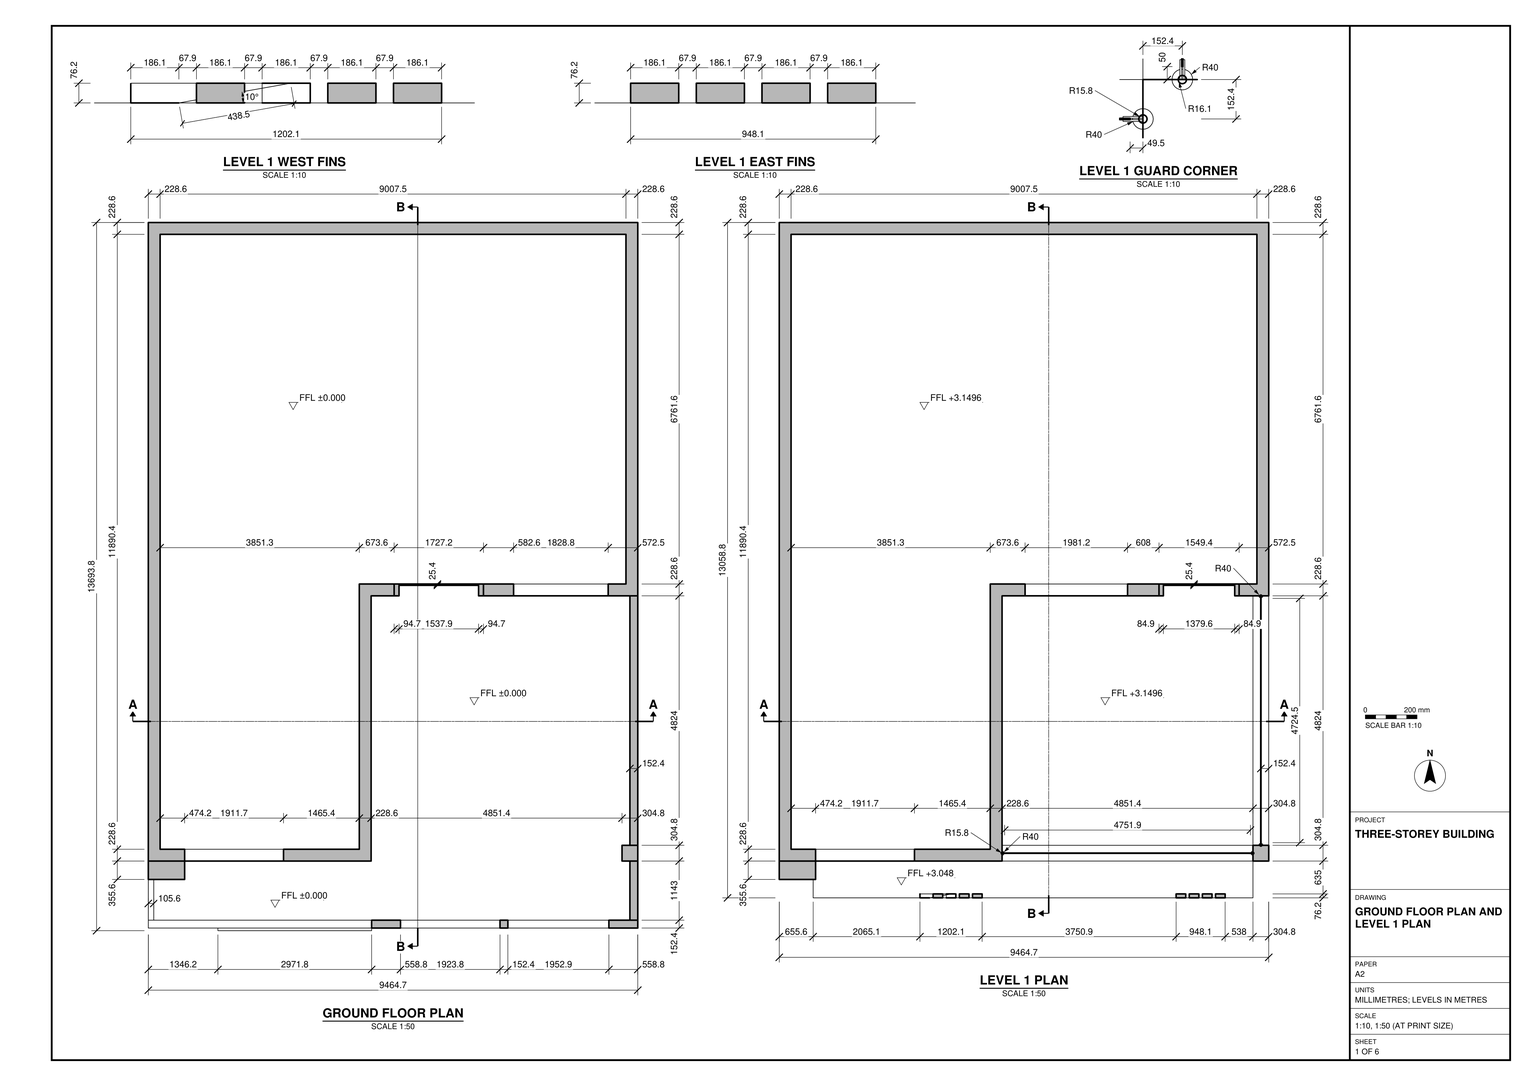
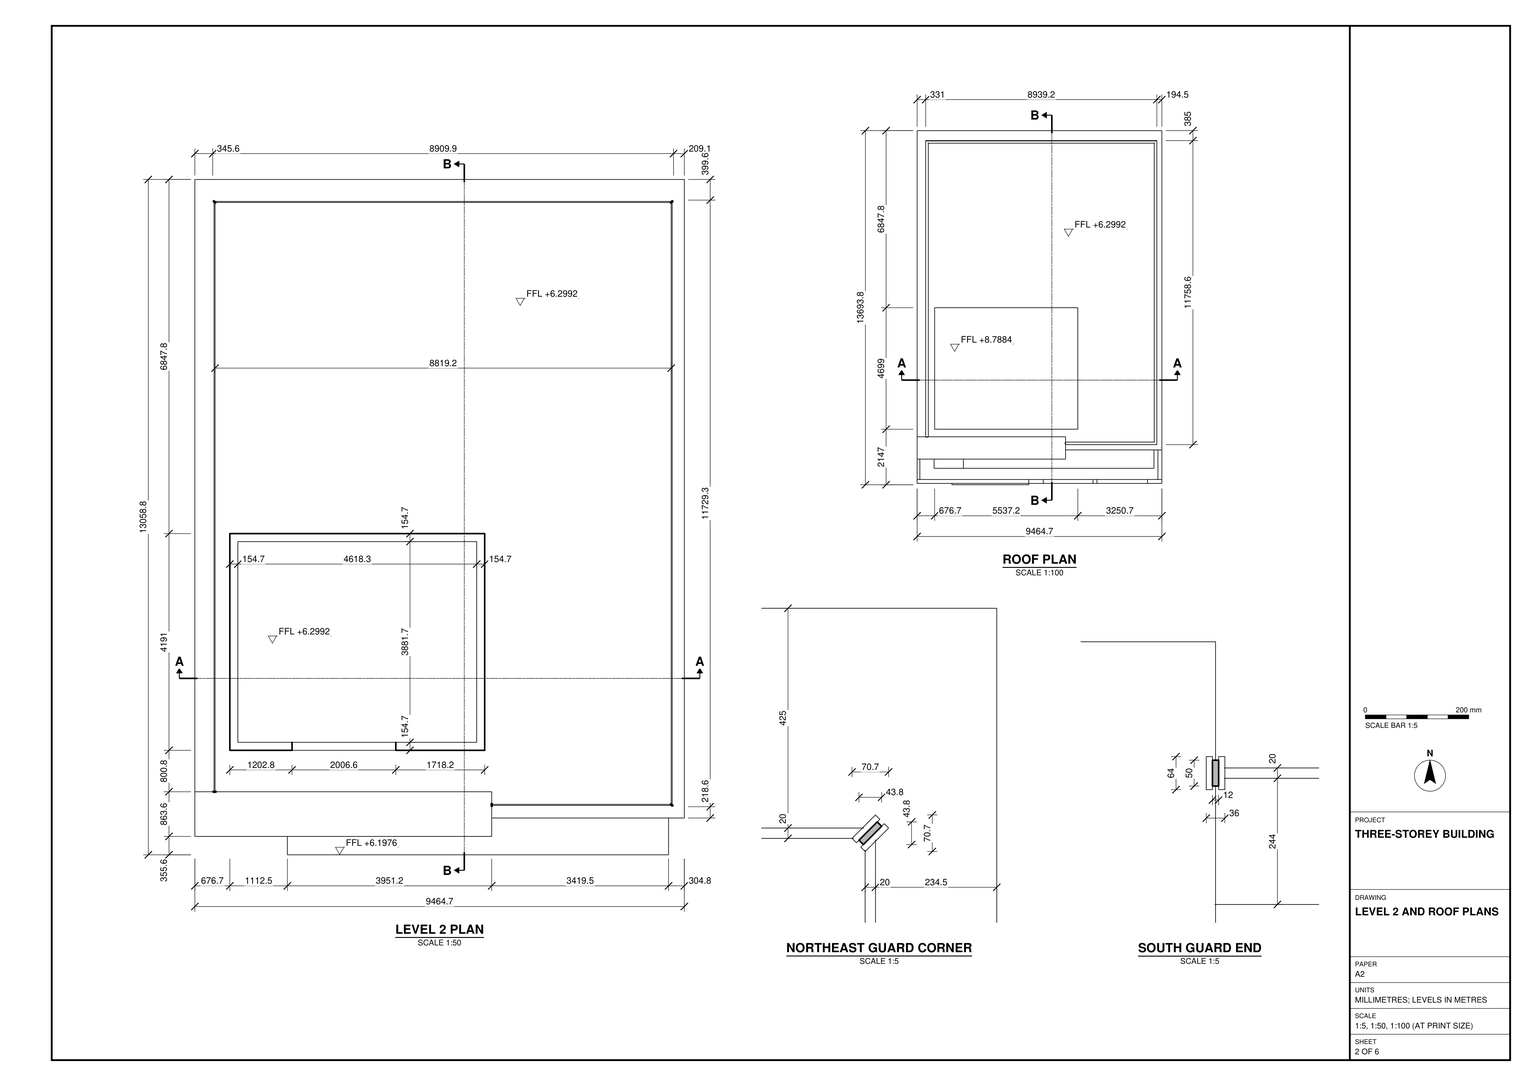
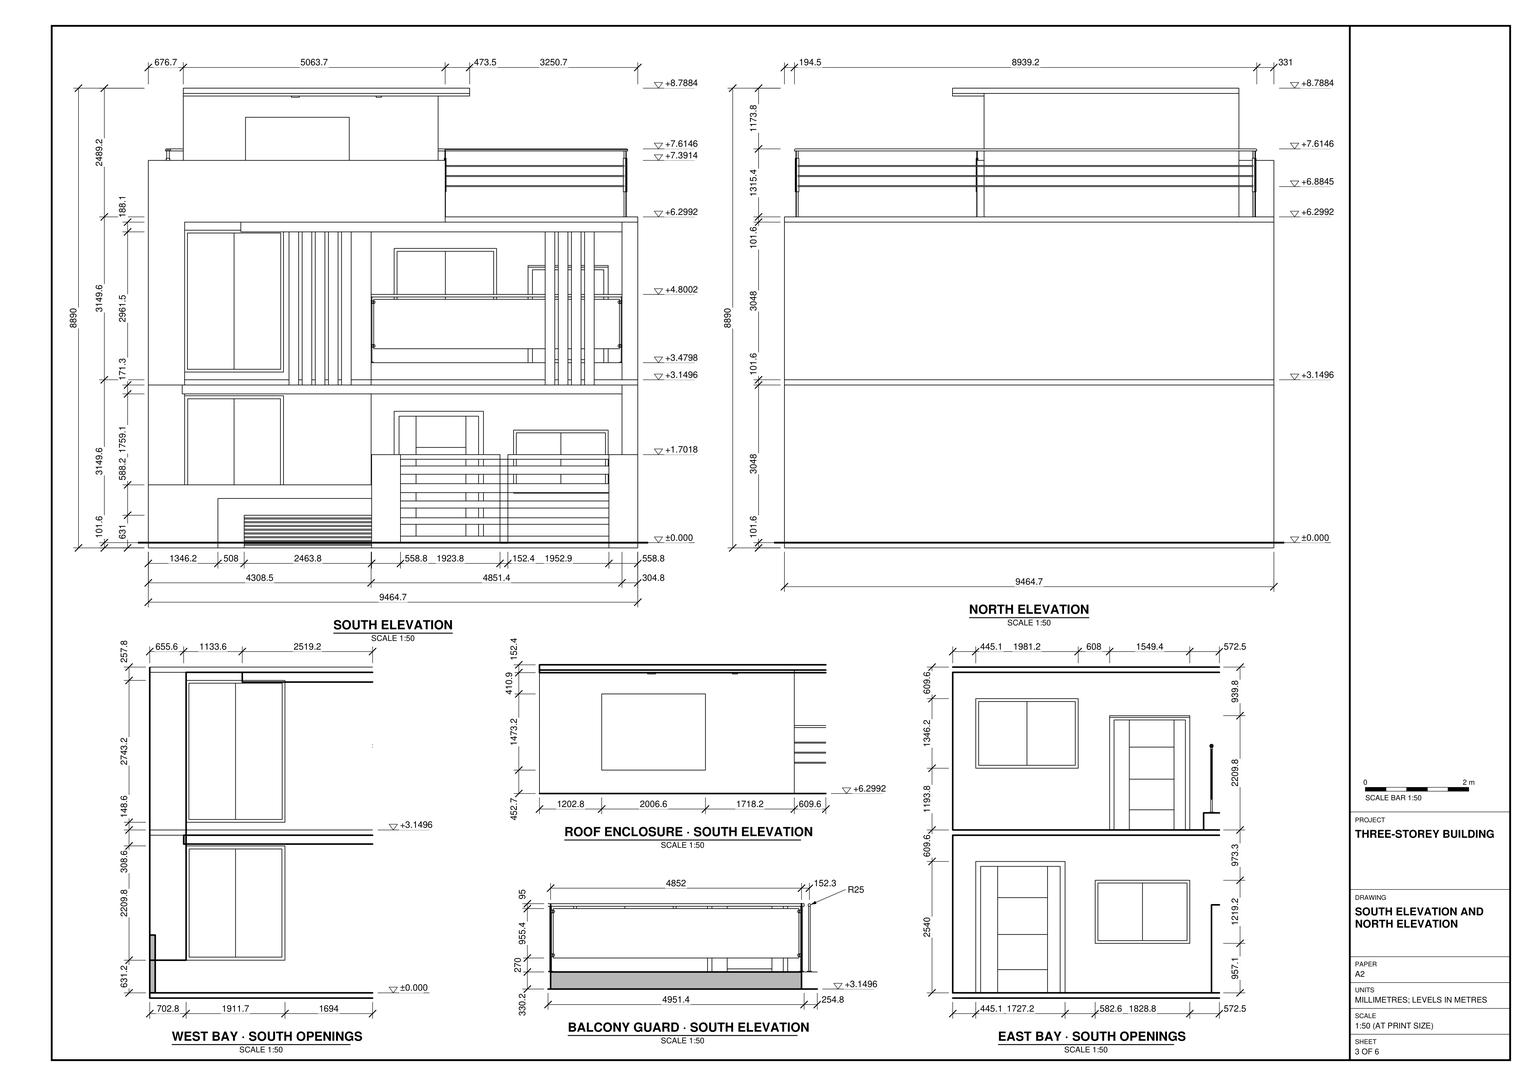
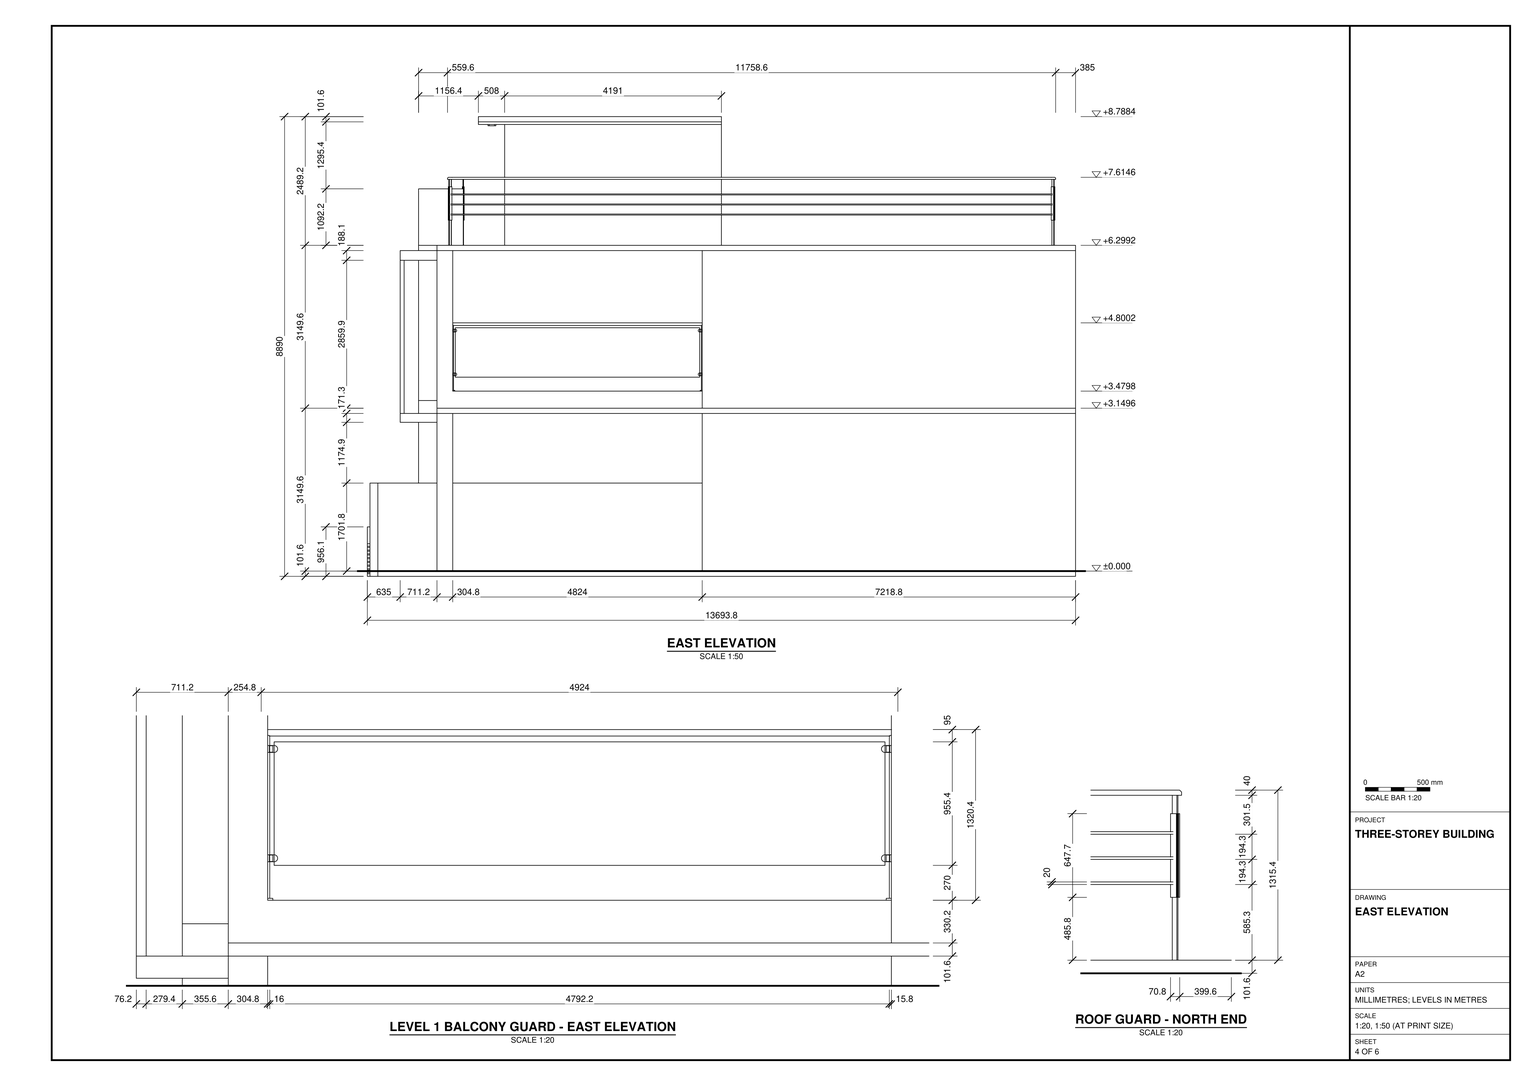
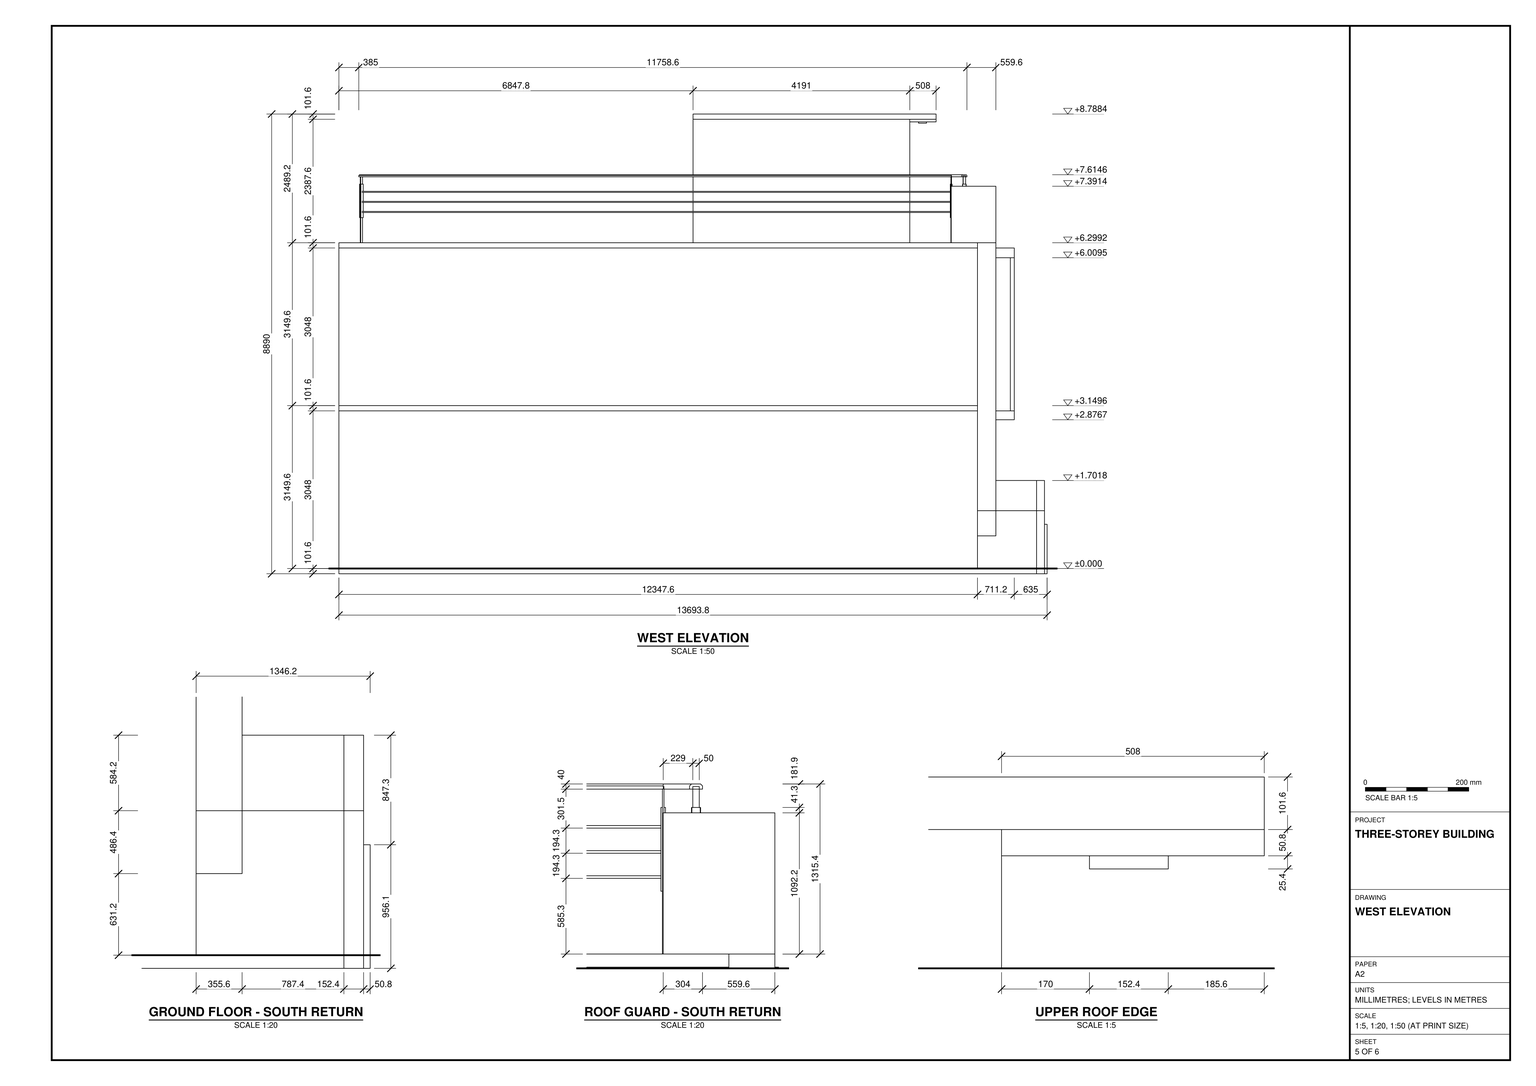
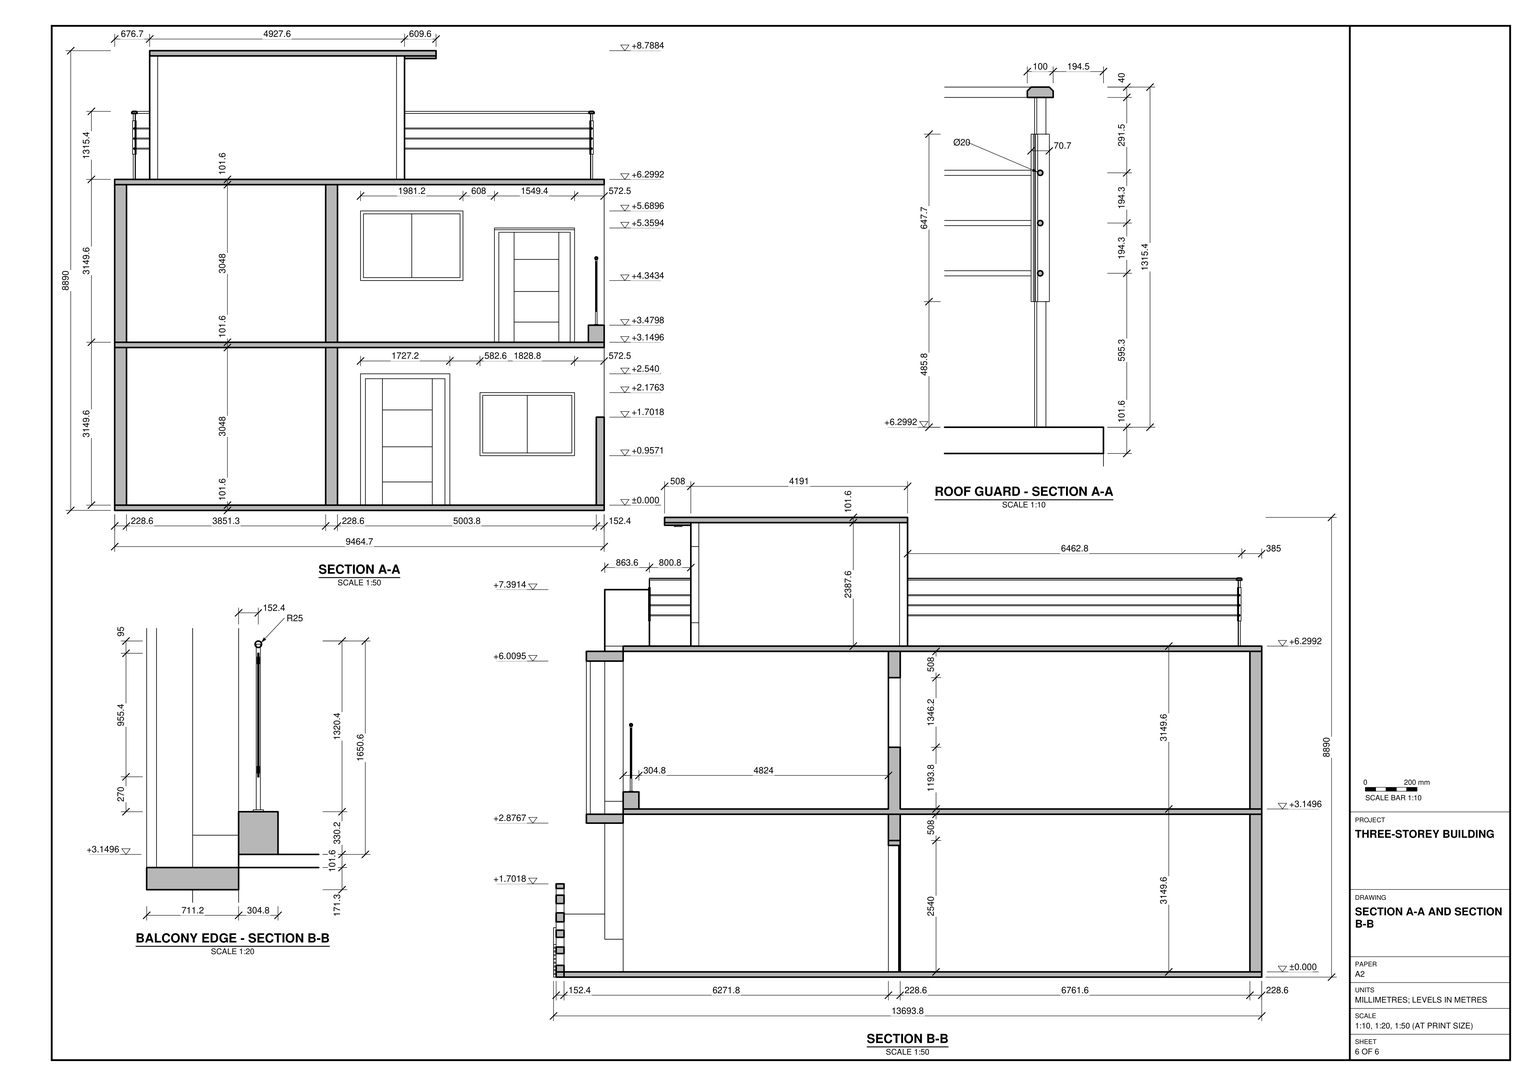
Build the three-storey building in SketchUp from task_files/diagram_01.pdf. Work in millimetres. The overall dimensions are 9464.7 mm east–west, 13693.8 mm north–south and 8890 mm high. Set the ground floor at 0 mm, level 1 at +3149.6 mm and level 2 at +6299.2 mm.

Use the floor plans to lay out the full-width north end, the projecting southwest bay and the recessed southeast bay. Model the floor slabs, the 228.6 mm main walls and the thinner walls where indicated. Keep the north wall uninterrupted by openings. On the south side, fit the tall paired window units in the west bay and the doors and windows in the recessed wall. Follow the elevations for their sill and head heights. Model the low front wall and horizontal slatted panels at ground level. At level 1, include the balcony guard, its corner return and the two distinct sets of vertical fins.

At level 2, form the open terrace with its parapet and rails. Place the smaller walled enclosure toward the southwest, with its south-facing opening and projecting flat roof. Keep walls, slabs, roof elements and each furniture or joinery piece shown in separate groups or components, and use components for repeated parts. Any decor or loose items shown may be represented by suitable library components. Save one SketchUp model as output_files/three_storey_building_with_a_balcony_and_roof_terrace.skp.

# SketchUp Ruby script. Lengths in millimetres.
U = 1.mm
M = Sketchup.active_model
def pt(a) = Geom::Point3d.new(a.map { |v| v * U })
def face(e, loops, mat)
  f = e.add_face(loops[0].map { |a| pt(a) })
  loops[1..].each { |l| e.add_face(l.map { |a| pt(a) }).erase! }
  f.material = f.back_material = mat if mat
  f
end
# faces: each face lists its corners as indices into pts; further lists are holes
def faces(e, pts, list, mat = nil) = list.each { |f| face(e, (f[0].is_a?(Array) ? f : [f]).map { |l| l.map { |i| pts[i] } }, mat) }
# xy, xz, yz: faces in a plane at the given z, y or x. An outline is a flat list of corners, or four numbers for a rectangle; further outlines are holes
def ring(l) = l.size == 4 ? [[l[0], l[1]], [l[2], l[1]], [l[2], l[3]], [l[0], l[3]]] : l.each_slice(2).to_a
def flat(e, list, mat, &to3) = list.each { |f| face(e, (f[0].is_a?(Array) ? f : [f]).map { |l| ring(l).map { |u, v| to3.(u, v) } }, mat) }
def xy(e, z, list, mat = nil) = flat(e, list, mat) { |x, y| [x, y, z] }
def xz(e, y, list, mat = nil) = flat(e, list, mat) { |x, z| [x, y, z] }
def yz(e, x, list, mat = nil) = flat(e, list, mat) { |y, z| [x, y, z] }
def lines(e, pts, list) = list.each { |a, b| e.add_line(pt(pts[a]), pt(pts[b])) }
# prism: a flat outline (further loops are holes) pulled along v
def prism(e, loops, v, mat = nil)
  f = face(e, loops, mat); d = Geom::Vector3d.new(v.map { |x| x * U })
  f.pushpull(f.normal.samedirection?(d) ? d.length : -d.length)
end
def box(e, o, s, mat = nil) = prism(e, [[o, [o[0] + s[0], o[1], o[2]], [o[0] + s[0], o[1] + s[1], o[2]], [o[0], o[1] + s[1], o[2]]]], [0, 0, s[2]], mat)
def at(x, y, z, deg = 0) = Geom::Transformation.translation(pt([x, y, z])) * Geom::Transformation.rotation(ORIGIN, Z_AXIS, deg.degrees)
def axes(o, x, y, z) = Geom::Transformation.new([*x, 0, *y, 0, *z, 0, *pt(o).to_a, 1])
def part(name) = M.definitions.add(name)
# library, detail: a bought-in or finely detailed component or shape, given as its bounding box
def library(name, o, s) = part(name).tap { |d| box(d.entities, o, s) }
def detail(e, o, s) = box(e.add_group.entities, o, s)
def put(e, d, t, mat = nil) = e.add_instance(d, t).tap { |i| i.material = mat if mat }
def group(e, t, mat = nil) = e.add_group.tap { |g| g.transformation = t; g.material = mat if mat }.entities
root = M.entities
M.materials.add("[Cladding Siding Tan]").color = [162, 126, 95]
M.materials.add("[Color B07]").color = [153, 38, 0]
M.materials.add("[Color C07]").color = [153, 76, 0]
M.materials.add("[Color E04]").color = [255, 255, 50]
M.materials.add("[Color M06]").color = [86, 86, 86]
M.materials.add("[Color M09]").color = [0, 0, 0]
M.materials.add("[Wood Veneer 01]").color = [120, 70, 37]
M.materials.add("[Wood Veneer 02]").color = [190, 128, 91]
c1 = library("Group\#4",[0,0,0],[4951.4,80,1320.4])
c2 = library("Group\#11",[0,0,0],[80,4924,1320.4])
c3 = library("Group\#7",[0,0,0],[8939.2,11758.6,730.1])
c4 = part("Ploe")
box(c4.entities,[5734.4,229,6400.8],[12,50,1295.4])
box(c4.entities,[5746.4,222,6886.6],[12,64,647.7],"[Wood Veneer 02]")
box(c4.entities,[5722.4,222,6886.6],[12,64,647.7],"[Wood Veneer 02]")
c5 = part("Group8\#1")
put(c5.entities,c4,at(0,0,0))
put(c5.entities,c4,at(5340.7,-3984.7,0,45))
put(c5.entities,c4,at(4981.5,15792.1,0,-45))
put(c5.entities,c4,at(4260.5,16151.3,0,-135))
put(c5.entities,c4,at(127,6248.4,0,-90))
c6 = part("Horizontal slat panel")
box(c6.entities,[0,-50.8,0],[2463.8,50.8,50.3])
box(c6.entities,[0,-50.8,-72.6],[2463.8,50.8,50.3])
box(c6.entities,[0,-50.8,-145.2],[2463.8,50.8,50.3])
box(c6.entities,[0,-50.8,-217.8],[2463.8,50.8,50.4])
box(c6.entities,[0,-50.8,-290.3],[2463.8,50.8,50.3])
box(c6.entities,[0,-50.8,-362.9],[2463.8,50.8,50.3])
box(c6.entities,[0,-50.8,-435.5],[2463.8,50.8,50.3])
box(c6.entities,[0,-50.8,-508.1],[2463.8,50.8,50.3])
box(c6.entities,[0,-50.8,-580.7],[2463.8,50.8,50.3])
c7 = part("Group\#10")
xy(c7.entities,0,[[0,0,0,228.6,1727.2,228.6,1727.2,0,1632.5,0,1632.5,203.2,94.7,203.2,94.7,0]],"[Wood Veneer 01]")
xy(c7.entities,2445.3,[[94.7,0,1632.5,203.2]],"[Wood Veneer 01]")
xy(c7.entities,2540,[[0,0,1727.2,228.6]],"[Wood Veneer 01]")
xz(c7.entities,0,[[0,0,94.7,0,94.7,2445.3,1632.5,2445.3,1632.5,0,1727.2,0,1727.2,2540,0,2540]],"[Wood Veneer 01]")
xz(c7.entities,203.2,[[94.7,0,423.7,2445.3],[423.7,0,1387.9,448.6],[1387.9,0,1632.5,2445.3],[423.7,448.6,1387.9,1128.7],[423.7,1128.7,1387.9,1841.3],
  [423.7,1841.3,1387.9,2445.3]],"[Wood Veneer 01]")
xz(c7.entities,228.6,[[0,0,1727.2,2540]],"[Wood Veneer 01]")
yz(c7.entities,0,[[0,0,228.6,2540]],"[Wood Veneer 01]")
yz(c7.entities,94.7,[[0,0,203.2,2445.3]],"[Wood Veneer 01]")
yz(c7.entities,1632.5,[[0,0,203.2,2445.3]],"[Wood Veneer 01]")
yz(c7.entities,1727.2,[[0,0,228.6,2540]],"[Wood Veneer 01]")
box(root,[3482.7,635,3149.6],[186.1,76.2,2961.5],"[Color M06]")
box(root,[3736.7,635,3149.6],[186.1,76.2,2961.5],"[Color M06]")
box(root,[7673.7,635,3149.6],[186.1,76.2,2961.5],"[Color M06]")
box(root,[7927.7,635,3149.6],[186.1,76.2,2961.5],"[Color M06]")
box(root,[8181.7,635,3149.6],[186.1,76.2,2961.5],"[Color M06]")
box(root,[8435.7,635,3149.6],[186.1,76.2,2961.5],"[Color M06]")
prism(root,[[[9464.7,1651,101.6],[9464.7,2870.2,101.6],[9464.7,6475,101.6],[9464.7,6475,1803.4],[9464.7,1651,1803.4]]],[-152.4,0,0])
xy(root,0,[[4318,50.8,8905.9,203.2],[8905.9,50.8,9464.7,203.2]])
xy(root,88.4,[[6800.6,50.8,6953,203.2]])
xy(root,100.3,[[4876.8,50.8,8905.9,203.2]])
xy(root,101.6,[[0,203.2,105.6,1346.2],[9312.3,203.2,9464.7,1346.2]])
xy(root,227.5,[[4876.8,50.8,8905.9,203.2]],"[Color M06]")
xy(root,455.6,[[4876.8,50.8,8905.9,203.2]],"[Color M06]")
xy(root,582.2,[[4876.8,50.8,8905.9,203.2]],"[Color M06]")
xy(root,732.8,[[0,990.6,702.8,1346.2]])
xy(root,770.3,[[4876.8,50.8,8905.9,203.2]],"[Color M06]")
xy(root,907.6,[[4876.8,50.8,8905.9,203.2]],"[Color M06]")
xy(root,1069.1,[[4876.8,50.8,8905.9,203.2]],"[Color M06]")
xy(root,1219.2,[[0,203.2,105.6,1346.2]])
xy(root,1242.2,[[4876.8,50.8,8905.9,203.2]],"[Color M06]")
xy(root,1423.5,[[4876.8,50.8,8905.9,203.2]],"[Color M06]")
xy(root,1584.5,[[4876.8,50.8,8905.9,203.2]],"[Color M06]")
xy(root,1714,[[4876.8,50.8,6800.6,203.2],[6953,50.8,8905.9,203.2]],"[Color M06]")
xy(root,1714,[[6800.6,50.8,6953,203.2]],"[Color M09]")
xy(root,1803.4,[[4318,50.8,4876.8,203.2],[8905.9,50.8,9464.7,203.2],[9312.3,203.2,9464.7,1346.2]])
xy(root,1803.4,[[4876.8,50.8,6800.6,203.2],[6953,50.8,8905.9,203.2]],"[Color M06]")
xy(root,3149.6,[[2720.7,635,2720.7,711.2,2974.7,711.2,2974.7,647,2906.8,635],[2974.7,635,2974.7,647,3160.8,679.8,3160.8,635],[3228.7,635,3228.7,691.8,3338.6,711.2,3414.8,711.2,3414.8,635],[2974.7,647,2974.7,711.2,3160.8,711.2,3160.8,679.8],[3160.8,679.8,3160.8,711.2,3228.7,711.2,3228.7,691.8],
  [3228.7,691.8,3228.7,711.2,3338.6,711.2]],"[Color M06]")
xy(root,6111.1,[[2720.7,635,2906.8,635,2974.7,647,2974.7,711.2,2720.7,711.2],[2974.7,635,3160.8,635,3160.8,679.8,2974.7,647],[3228.7,635,3414.8,635,3414.8,711.2,3338.6,711.2,3228.7,691.8],[2974.7,647,3160.8,679.8,3160.8,711.2,2974.7,711.2],[3160.8,679.8,3228.7,691.8,3228.7,711.2,3160.8,711.2],
  [3228.7,691.8,3338.6,711.2,3228.7,711.2]],"[Color M06]")
xy(root,6299.2,[[702.8,990.6,5740.4,1346.2]])
xy(root,6400.8,[[0,1346.2,5740.4,1854.2],[[676.7,2655,5604.3,6846],[831.4,2809.6,5449.7,6691.3]],[831.4,2809.6,5449.7,6691.3]])
xy(root,6853.5,[[1879.5,2655,3886.1,2809.6]])
xy(root,7493,[[0,990.6,5740.4,1854.2]])
xy(root,8326.7,[[1879.5,2655,3886.1,2809.6]])
xy(root,8712.2,[[2843.1,2332.6,2823.4,2335.2,2805,2342.8,2789.2,2354.9,2777.1,2370.7,2769.5,2389.1,2766.9,2408.8,2769.5,2428.5,2777.1,2446.9,2789.2,2462.7,2805,2474.8,2823.4,2482.4,2843.1,2485,2862.8,2482.4,2881.2,2474.8,2897,2462.7,2909.1,2446.9,2916.7,2428.5,2919.3,2408.8,2916.7,2389.1,2909.1,2370.7,2897,2354.9,2881.2,2342.8,2862.8,2335.2],[4456.2,2356.9,4443,2358.6,4430.8,2363.7,4420.3,2371.8,4412.2,2382.3,4407.1,2394.6,4405.4,2407.7,4407.1,2420.9,4412.2,2433.1,4420.3,2443.6,4430.8,2451.7,4443,2456.8,4456.2,2458.5,4469.3,2456.8,4481.6,2451.7,4492.1,2443.6,4500.2,2433.1,4505.2,2420.9,4507,2407.7,4505.2,2394.6,4500.2,2382.3,4492.1,2371.8,4481.6,2363.7,4469.3,2358.6]],"[Color E04]")
xy(root,8737.6,[[[676.7,2147,676.7,2655,5604.3,2655,5604.3,6846,6213.9,6846,6213.9,2147],[2843.1,2332.6,2862.8,2335.2,2881.2,2342.8,2897,2354.9,2909.1,2370.7,2916.7,2389.1,2919.3,2408.8,2916.7,2428.5,2909.1,2446.9,2897,2462.7,2881.2,2474.8,2862.8,2482.4,2843.1,2485,2823.4,2482.4,2805,2474.8,2789.2,2462.7,2777.1,2446.9,2769.5,2428.5,2766.9,2408.8,2769.5,2389.1,2777.1,2370.7,2789.2,2354.9,2805,2342.8,2823.4,2335.2],[4456.2,2356.9,4469.3,2358.6,4481.6,2363.7,4492.1,2371.8,4500.2,2382.3,4505.2,2394.6,4507,2407.7,4505.2,2420.9,4500.2,2433.1,4492.1,2443.6,4481.6,2451.7,4469.3,2456.8,4456.2,2458.5,4443,2456.8,4430.8,2451.7,4420.3,2443.6,4412.2,2433.1,4407.1,2420.9,4405.4,2407.7,4407.1,2394.6,4412.2,2382.3,4420.3,2371.8,4430.8,2363.7,4443,2358.6]]],"[Color B07]")
xy(root,8788.4,[[676.7,2147,6213.9,2147,6213.9,6846,5604.3,6846,5604.3,2655,676.7,2655],[676.7,2655,5604.3,6846]])
xy(root,8890,[[676.7,2147,6213.9,6846]])
xz(root,50.8,[[4318,0,8905.9,0,8905.9,100.3,6953,100.3,6953,88.4,6800.6,88.4,6800.6,100.3,4876.8,100.3,4876.8,1803.4,4318,1803.4],[8905.9,0,9464.7,1803.4],[6800.6,88.4,6953,100.3]])
xz(root,50.8,[[4876.8,100.3,6800.6,227.5],[6953,100.3,8905.9,227.5],[4876.8,455.6,6800.6,582.2],[6953,455.6,8905.9,582.2],[4876.8,770.3,6800.6,907.6],
  [6953,770.3,8905.9,907.6],[4876.8,1069.1,6800.6,1242.2],[6953,1069.1,8905.9,1242.2],[4876.8,1423.5,6800.6,1584.5],[6953,1423.5,8905.9,1584.5],
  [4876.8,1714,6800.6,1803.4],[6953,1714,8905.9,1803.4]],"[Color M06]")
xz(root,50.8,[[6800.6,100.3,6953,227.5],[6800.6,227.5,6953,455.6],[6800.6,455.6,6953,582.2],[6800.6,582.2,6953,770.3],[6800.6,770.3,6953,907.6],
  [6800.6,907.6,6953,1069.1],[6800.6,1069.1,6953,1242.2],[6800.6,1242.2,6953,1423.5],[6800.6,1423.5,6953,1584.5],[6800.6,1584.5,6953,1714]],"[Color M09]")
xz(root,203.2,[[4318,0,4318,1803.4,4876.8,1803.4,4876.8,100.3,6800.6,100.3,6800.6,88.4,6953,88.4,6953,100.3,8905.9,100.3,8905.9,0],[8905.9,0,8905.9,1803.4,9312.3,1803.4,9312.3,101.6,9464.7,101.6,9464.7,0],[6800.6,88.4,6953,100.3],[4876.8,100.3,6800.6,227.5],[6800.6,100.3,6953,227.5],
  [6953,100.3,8905.9,227.5],[0,101.6,105.6,1219.2],[9312.3,101.6,9464.7,1803.4],[6800.6,227.5,6953,455.6],[4876.8,455.6,6800.6,582.2],
  [6800.6,455.6,6953,582.2],[6953,455.6,8905.9,582.2],[6800.6,582.2,6953,770.3],[4876.8,770.3,6800.6,907.6],[6800.6,770.3,6953,907.6],
  [6953,770.3,8905.9,907.6],[6800.6,907.6,6953,1069.1],[4876.8,1069.1,6800.6,1242.2],[6800.6,1069.1,6953,1242.2],[6953,1069.1,8905.9,1242.2],
  [6800.6,1242.2,6953,1423.5],[4876.8,1423.5,6800.6,1584.5],[6800.6,1423.5,6953,1584.5],[6953,1423.5,8905.9,1584.5],[6800.6,1584.5,6953,1714],
  [4876.8,1714,6800.6,1803.4],[6953,1714,8905.9,1803.4]])
xz(root,635,[[2720.7,3149.6,2906.8,6111.1],[2974.7,3149.6,3160.8,6111.1],[3228.7,3149.6,3414.8,6111.1]],"[Color M06]")
xz(root,711.2,[[2974.7,3149.6,3160.8,6111.1],[3228.7,3149.6,3338.6,6111.1],[3338.6,3149.6,3414.8,6111.1]],"[Color M06]")
xz(root,990.6,[[0,732.8,702.8,3149.6]])
xz(root,990.6,[[0,3149.6,702.8,3149.6,702.8,6299.2,5740.4,6299.2,5740.4,7493,0,7493]],"[Cladding Siding Tan]")
xz(root,1346.2,[[0,101.6,105.6,732.8],[9312.3,101.6,9464.7,1803.4],[0,732.8,105.6,1219.2],[105.6,732.8,105.6,1219.2,0,1219.2,0,6400.8,5740.4,6400.8,5740.4,6299.2,702.8,6299.2,702.8,732.8],[761.8,791.8,1658.7,2883.6],
  [1658.7,791.8,2555.5,2883.6],[756.8,3453.8,1658.7,6089.1],[1658.7,3453.8,2560.6,6089.1]])
xz(root,1346.2,[[[702.8,732.8,2614.5,2942.6],[761.8,791.8,2555.5,2883.6]],[[702.8,3399.8,2614.5,6143],[756.8,3453.8,2560.6,6089.1]]],"[Color M09]")
xz(root,1854.2,[[0,6400.8,5740.4,7493]])
xz(root,2147,[[676.7,8737.6,6213.9,8788.4],[676.7,8788.4,6213.9,8890]])
xz(root,2655,[[[676.7,6400.8,5604.3,8737.6],[1879.5,6853.5,3886.1,8326.7]],[676.7,8737.6,5604.3,8788.4]])
xz(root,6475,[[7115.9,1111.2,7977.8,2225.4],[7977.8,1111.2,8839.6,2225.4]])
xz(root,6475,[[[7063.4,1058.7,8892.2,2277.9],[7115.9,1111.2,8839.6,2225.4]]],"[Color C07]")
xz(root,6846,[[676.7,6400.8,5604.3,8788.4],[5604.3,8737.6,6213.9,8788.4],[676.7,8788.4,6213.9,8890]])
yz(root,0,[[203.2,101.6,203.2,1219.2,990.6,1219.2,990.6,732.8,1346.2,732.8,1346.2,101.6],[990.6,732.8,1346.2,1219.2],[990.6,1219.2,1346.2,6400.8],[990.6,6400.8,1854.2,7493]])
yz(root,105.6,[[203.2,101.6,1346.2,1219.2]])
yz(root,676.7,[[2655,6400.8,6846,8788.4],[2147,8737.6,2655,8788.4],[2147,8788.4,6846,8890]])
yz(root,702.8,[[990.6,732.8,1346.2,3399.8],[990.6,3399.8,1346.2,6299.2]])
yz(root,1879.5,[[2655,6853.5,2809.6,8326.7]])
yz(root,2720.7,[[635,3149.6,711.2,6111.1]],"[Color M06]")
yz(root,2974.7,[[635,3149.6,711.2,6111.1]],"[Color M06]")
yz(root,3160.8,[[635,3149.6,711.2,6111.1]],"[Color M06]")
yz(root,3414.8,[[635,3149.6,711.2,6111.1]],"[Color M06]")
yz(root,3886.1,[[2655,6853.5,2809.6,8326.7]])
yz(root,4318,[[50.8,0,203.2,1803.4]])
yz(root,4876.8,[[50.8,100.3,203.2,227.5],[50.8,227.5,203.2,455.6],[50.8,455.6,203.2,582.2],[50.8,582.2,203.2,770.3],[50.8,770.3,203.2,907.6],
  [50.8,907.6,203.2,1069.1],[50.8,1069.1,203.2,1242.2],[50.8,1242.2,203.2,1423.5],[50.8,1423.5,203.2,1584.5],[50.8,1584.5,203.2,1714],
  [50.8,1714,203.2,1803.4]])
yz(root,5604.3,[[2655,6400.8,6846,8737.6],[2655,8737.6,6846,8788.4]])
yz(root,5740.4,[[990.6,6299.2,1346.2,6400.8],[990.6,6400.8,1854.2,7493]])
yz(root,6213.9,[[2147,8737.6,6846,8788.4],[2147,8788.4,6846,8890]])
yz(root,6800.6,[[50.8,88.4,203.2,1714]])
yz(root,6800.6,[[50.8,1714,203.2,1803.4]],"[Color M06]")
yz(root,6953,[[50.8,88.4,203.2,1714]])
yz(root,6953,[[50.8,1714,203.2,1803.4]],"[Color M06]")
yz(root,8905.9,[[50.8,100.3,203.2,227.5],[50.8,227.5,203.2,455.6],[50.8,455.6,203.2,582.2],[50.8,582.2,203.2,770.3],[50.8,770.3,203.2,907.6],
  [50.8,907.6,203.2,1069.1],[50.8,1069.1,203.2,1242.2],[50.8,1242.2,203.2,1423.5],[50.8,1423.5,203.2,1584.5],[50.8,1584.5,203.2,1714],
  [50.8,1714,203.2,1803.4]])
yz(root,9312.3,[[203.2,101.6,1346.2,1803.4]])
yz(root,9464.7,[[50.8,0,203.2,1803.4],[203.2,101.6,1346.2,1803.4]])
p = [[2843.1,2332.6,8737.6],[2823.4,2335.2,8737.6],[2823.4,2335.2,8712.2],[2843.1,2332.6,8712.2],[2862.8,2335.2,8737.6],[2862.8,2335.2,8712.2],
  [2805,2342.8,8737.6],[2805,2342.8,8712.2],[2881.2,2342.8,8737.6],[2881.2,2342.8,8712.2],[2789.2,2354.9,8737.6],[2789.2,2354.9,8712.2],
  [2897,2354.9,8737.6],[2897,2354.9,8712.2],[2777.1,2370.7,8737.6],[2777.1,2370.7,8712.2],[2909.1,2370.7,8737.6],[2909.1,2370.7,8712.2],
  [4456.2,2356.9,8737.6],[4443,2358.6,8737.6],[4443,2358.6,8712.2],[4456.2,2356.9,8712.2],[4469.3,2358.6,8737.6],[4469.3,2358.6,8712.2],
  [4430.8,2363.7,8737.6],[4430.8,2363.7,8712.2],[4481.6,2363.7,8737.6],[4481.6,2363.7,8712.2],[4420.3,2371.8,8737.6],[4420.3,2371.8,8712.2],
  [4492.1,2371.8,8737.6],[4492.1,2371.8,8712.2],[2769.5,2389.1,8737.6],[2769.5,2389.1,8712.2],[2916.7,2389.1,8737.6],[2916.7,2389.1,8712.2],
  [4412.2,2382.3,8737.6],[4412.2,2382.3,8712.2],[4500.2,2382.3,8737.6],[4500.2,2382.3,8712.2],[4407.1,2394.6,8737.6],[4407.1,2394.6,8712.2],
  [4505.2,2394.6,8737.6],[4505.2,2394.6,8712.2],[2766.9,2408.8,8737.6],[2766.9,2408.8,8712.2],[2919.3,2408.8,8737.6],[2919.3,2408.8,8712.2],
  [4405.4,2407.7,8737.6],[4405.4,2407.7,8712.2],[4507,2407.7,8737.6],[4507,2407.7,8712.2],[4407.1,2420.9,8737.6],[4407.1,2420.9,8712.2],
  [4505.2,2420.9,8737.6],[4505.2,2420.9,8712.2],[2769.5,2428.5,8737.6],[2769.5,2428.5,8712.2],[2916.7,2428.5,8737.6],[2916.7,2428.5,8712.2],
  [4412.2,2433.1,8737.6],[4412.2,2433.1,8712.2],[4500.2,2433.1,8737.6],[4500.2,2433.1,8712.2],[2777.1,2446.9,8737.6],[2777.1,2446.9,8712.2],
  [2909.1,2446.9,8737.6],[2909.1,2446.9,8712.2],[4420.3,2443.6,8737.6],[4420.3,2443.6,8712.2],[4492.1,2443.6,8737.6],[4492.1,2443.6,8712.2],
  [4430.8,2451.7,8737.6],[4430.8,2451.7,8712.2],[4481.6,2451.7,8737.6],[4481.6,2451.7,8712.2],[2789.2,2462.7,8737.6],[2789.2,2462.7,8712.2],
  [2897,2462.7,8737.6],[2897,2462.7,8712.2],[4443,2456.8,8737.6],[4443,2456.8,8712.2],[4469.3,2456.8,8737.6],[4469.3,2456.8,8712.2],
  [4456.2,2458.5,8737.6],[4456.2,2458.5,8712.2],[2805,2474.8,8737.6],[2805,2474.8,8712.2],[2881.2,2474.8,8737.6],[2881.2,2474.8,8712.2],
  [2823.4,2482.4,8737.6],[2823.4,2482.4,8712.2],[2862.8,2482.4,8737.6],[2862.8,2482.4,8712.2],[2843.1,2485,8737.6],[2843.1,2485,8712.2],
  [5449.7,6691.3,6400.8],[5449.7,6691.3,8788.4],[831.4,6691.3,6400.8],[831.4,6691.3,8788.4],[5449.7,2809.6,6400.8],[5449.7,2809.6,8788.4],
  [831.4,2809.6,6400.8],[831.4,2809.6,8788.4]]
faces(root,p,[[0,1,2,3],[4,0,3,5],[1,6,7,2],[8,4,5,9],[6,10,11,7],[12,8,9,13],[10,14,15,11],[16,12,13,17],
  [18,19,20,21],[22,18,21,23],[19,24,25,20],[26,22,23,27],[24,28,29,25],[30,26,27,31],[14,32,33,15],[34,16,17,35],
  [28,36,37,29],[38,30,31,39],[36,40,41,37],[42,38,39,43],[32,44,45,33],[46,34,35,47],[40,48,49,41],[50,42,43,51],
  [48,52,53,49],[54,50,51,55],[44,56,57,45],[58,46,47,59],[52,60,61,53],[62,54,55,63],[56,64,65,57],[66,58,59,67],
  [60,68,69,61],[70,62,63,71],[68,72,73,69],[74,70,71,75],[64,76,77,65],[78,66,67,79],[72,80,81,73],[82,74,75,83],
  [80,84,85,81],[84,82,83,85],[76,86,87,77],[88,78,79,89],[86,90,91,87],[92,88,89,93],[90,94,95,91],[94,92,93,95]],"[Color E04]")
lines(root,p,[[96,97],[98,99],[100,101],[102,103]])
g1 = group(root,at(0,1346.2,0))
xy(g1,0,[[0,-1143,9464.7,12347.6]])
xy(g1,101.6,[[0,-1143,9464.7,-1143,9464.7,5128.8,6480.7,5128.8,6480.7,5357.4,9236.1,5357.4,9236.1,12119,228.6,12119,228.6,228.6,4079.9,228.6,4079.9,5357.4,4753.5,5357.4,4753.5,5128.8,4308.5,5128.8,4308.5,0,0,0],[0,0,0,12347.6,9464.7,12347.6,9464.7,5128.8,6480.7,5128.8,6480.7,5357.4,9236.1,5357.4,9236.1,12119,228.6,12119,228.6,228.6,4079.9,228.6,4079.9,5357.4,4753.5,5357.4,4753.5,5128.8,4308.5,5128.8,4308.5,0]])
xy(g1,732.8,[[702.8,0,2614.5,228.6]])
xy(g1,1058.7,[[7063.4,5128.8,8892.2,5357.4]])
xy(g1,2277.9,[[7063.4,5128.8,8892.2,5357.4]])
xy(g1,2641.6,[[4753.5,5128.8,6480.7,5357.4]])
xy(g1,2942.6,[[702.8,0,2614.5,228.6]])
xy(g1,3149.6,[[[0,0,4308.5,0,4308.5,5128.8,9464.7,5128.8,9464.7,12347.6,0,12347.6],[228.6,228.6,228.6,12119,9236.1,12119,9236.1,5357.4,4079.9,5357.4,4079.9,228.6]]])
xz(g1,-1143,[[0,0,4308.5,101.6],[4308.5,0,9464.7,101.6]])
xz(g1,0,[[[0,101.6,4308.5,3149.6],[702.8,732.8,2614.5,2942.6]]])
xz(g1,228.6,[[[228.6,101.6,4079.9,3149.6],[702.8,732.8,2614.5,2942.6]]])
xz(g1,5128.8,[[[4308.5,101.6,4753.5,101.6,4753.5,2641.6,6480.7,2641.6,6480.7,101.6,9464.7,101.6,9464.7,3149.6,4308.5,3149.6],[7063.4,1058.7,8892.2,2277.9]]])
xz(g1,5357.4,[[[4079.9,101.6,4079.9,3149.6,9236.1,3149.6,9236.1,101.6,6480.7,101.6,6480.7,2641.6,4753.5,2641.6,4753.5,101.6],[7063.4,1058.7,8892.2,2277.9]]])
xz(g1,12119,[[228.6,101.6,9236.1,3149.6]])
xz(g1,12347.6,[[0,0,9464.7,101.6],[0,101.6,9464.7,3149.6]])
yz(g1,0,[[-1143,0,12347.6,101.6],[0,101.6,12347.6,3149.6]])
yz(g1,228.6,[[228.6,101.6,12119,3149.6]])
yz(g1,702.8,[[0,732.8,228.6,2942.6]])
yz(g1,2614.5,[[0,732.8,228.6,2942.6]])
yz(g1,4079.9,[[228.6,101.6,5357.4,3149.6]])
yz(g1,4308.5,[[0,101.6,5128.8,3149.6]])
yz(g1,4753.5,[[5128.8,101.6,5357.4,2641.6]])
yz(g1,6480.7,[[5128.8,101.6,5357.4,2641.6]])
yz(g1,7063.4,[[5128.8,1058.7,5357.4,2277.9]])
yz(g1,8892.2,[[5128.8,1058.7,5357.4,2277.9]])
yz(g1,9236.1,[[5357.4,101.6,12119,3149.6]])
yz(g1,9464.7,[[-1143,0,12347.6,101.6],[5128.8,101.6,12347.6,3149.6]])
g2 = group(root,at(0,1346.2,3149.6))
xy(g2,0,[[0,0,9464.7,12347.6]])
xy(g2,101.6,[[0,0,0,12347.6,9464.7,12347.6,9464.7,5128.8,8892.2,5128.8,8892.2,5357.4,9236.1,5357.4,9236.1,12119,228.6,12119,228.6,228.6,4079.9,228.6,4079.9,5357.4,4753.5,5357.4,4753.5,5128.8,4308.5,5128.8,4308.5,0],[4308.5,0,9464.7,0,9464.7,5128.8,8892.2,5128.8,8892.2,5357.4,9236.1,5357.4,9236.1,12119,228.6,12119,228.6,228.6,4079.9,228.6,4079.9,5357.4,7342.8,5357.4,7342.8,5128.8,4308.5,5128.8],[6480.7,5128.8,7342.8,5357.4]])
xy(g2,250.2,[[702.8,0,2614.5,228.6]])
xy(g2,1295.4,[[4753.5,5128.8,6734.7,5357.4]])
xy(g2,2277.9,[[7342.8,5128.8,8892.2,5357.4]])
xy(g2,2641.6,[[4753.5,5128.8,6734.7,5357.4]])
xy(g2,2993.4,[[702.8,0,2614.5,228.6]])
xy(g2,3149.6,[[[0,0,4308.5,0,4308.5,5128.8,9464.7,5128.8,9464.7,12347.6,0,12347.6],[228.6,228.6,228.6,12119,9236.1,12119,9236.1,5357.4,4079.9,5357.4,4079.9,228.6]]])
xz(g2,0,[[0,0,4308.5,101.6],[4308.5,0,9464.7,101.6],[[0,101.6,4308.5,3149.6],[702.8,250.2,2614.5,2993.4]]])
xz(g2,228.6,[[[228.6,101.6,4079.9,3149.6],[702.8,250.2,2614.5,2993.4]]])
xz(g2,5128.8,[[[4308.5,101.6,7342.8,101.6,7342.8,2277.9,8892.2,2277.9,8892.2,101.6,9464.7,101.6,9464.7,3149.6,4308.5,3149.6],[4753.5,1295.4,6734.7,2641.6]],[4810.1,1351.9,5744.1,2585.1],[5744.1,1351.9,6678.2,2585.1]])
xz(g2,5128.8,[[[4753.5,1295.4,6734.7,2641.6],[4810.1,1351.9,6678.2,2585.1]]],"[Color C07]")
xz(g2,5357.4,[[4079.9,101.6,4079.9,3149.6,9236.1,3149.6,9236.1,101.6,8892.2,101.6,8892.2,2277.9,7342.8,2277.9,7342.8,101.6,6480.7,101.6,6480.7,1295.4,6734.7,1295.4,6734.7,2641.6,4753.5,2641.6,4753.5,101.6],[4753.5,101.6,6480.7,1295.4]])
xz(g2,12119,[[228.6,101.6,9236.1,3149.6]])
xz(g2,12347.6,[[0,0,9464.7,101.6],[0,101.6,9464.7,3149.6]])
yz(g2,0,[[0,0,12347.6,101.6],[0,101.6,12347.6,3149.6]])
yz(g2,228.6,[[228.6,101.6,12119,3149.6]])
yz(g2,702.8,[[0,250.2,228.6,2993.4]])
yz(g2,2614.5,[[0,250.2,228.6,2993.4]])
yz(g2,4079.9,[[228.6,101.6,5357.4,3149.6]])
yz(g2,4308.5,[[0,101.6,5128.8,3149.6]])
yz(g2,4753.5,[[5128.8,1295.4,5357.4,2641.6]])
yz(g2,6734.7,[[5128.8,1295.4,5357.4,2641.6]])
yz(g2,7342.8,[[5128.8,101.6,5357.4,2277.9]])
yz(g2,8892.2,[[5128.8,101.6,5357.4,2277.9]])
yz(g2,9236.1,[[5357.4,101.6,12119,3149.6]])
yz(g2,9464.7,[[0,0,12347.6,101.6],[5128.8,101.6,12347.6,3149.6]])
g3 = group(root,at(0,1346.2,6299.2))
box(g3,[0,0,0],[9464.7,12347.6,101.6])
put(root,c1,at(4258.5,1458.6,3581.4))
g4 = group(root,at(2551.2,660.4,3251.2))
xy(g4,0,[[6608.6,685.8,6913.4,5814.6]])
xy(g4,330.2,[[1757.2,685.8,6608.6,990.6],[6608.6,990.6,6913.4,5814.6]])
xy(g4,2859.9,[[-762,-25.4,6608.6,685.8]])
xy(g4,3048,[[-762,-25.4,6608.6,685.8],[6608.6,685.8,6913.4,990.6]])
xz(g4,-25.4,[[-762,2859.9,6608.6,3048]])
xz(g4,685.8,[[1757.2,0,6608.6,330.2],[6608.6,0,6913.4,3048],[-762,2859.9,6608.6,3048]])
xz(g4,990.6,[[1757.2,0,6608.6,330.2],[6608.6,330.2,6913.4,3048]])
xz(g4,5814.6,[[6608.6,0,6913.4,330.2]])
yz(g4,-762,[[-25.4,2859.9,685.8,3048]])
yz(g4,1757.2,[[685.8,0,990.6,330.2]])
yz(g4,6608.6,[[685.8,0,990.6,330.2],[990.6,0,5814.6,330.2],[685.8,330.2,990.6,3048],[-25.4,2859.9,685.8,3048]])
yz(g4,6913.4,[[685.8,0,5814.6,0,5814.6,330.2,990.6,330.2,990.6,3048,685.8,3048]])
put(g4,c2,at(6721,940.6,330.2))
g5 = group(root,at(2154.2,635,101.6))
xy(g5,0,[[7005.6,711.2,7310.4,1016]])
xy(g5,2876.7,[[-1498.6,0,7005.6,711.2]])
xy(g5,3048,[[-1498.6,0,7005.6,711.2],[7005.6,711.2,7310.4,1016]])
xz(g5,0,[[-1498.6,2876.7,7005.6,3048]])
xz(g5,711.2,[[7005.6,0,7310.4,3048],[-1498.6,2876.7,7005.6,3048]])
xz(g5,1016,[[7005.6,0,7310.4,3048]])
yz(g5,-1498.6,[[0,2876.7,711.2,3048]])
yz(g5,7005.6,[[711.2,0,1016,3048],[0,2876.7,711.2,3048]])
yz(g5,7310.4,[[711.2,0,1016,3048]])
g6 = group(root,at(331,1550.2,6400.8))
put(g6,c3,at(0,0,585.3))
put(g6,c5,at(-331,-204,-6400.8))
g7 = group(root,at(0,50.8,0))
xy(g7,0,[[1346.2,-50.8,1346.2,0,0,0,0,152.4,4318,152.4,4318,0,1854.2,0,1854.2,-50.8]])
xy(g7,631,[[1854.2,-50.8,4318,0]])
xy(g7,956.1,[[1346.2,-50.8,4318,0]],"[Color M06]")
xy(g7,1219.2,[[0,0,4318,152.4]])
xz(g7,-50.8,[[1346.2,0,1854.2,0,1854.2,631,4318,631,4318,956.1,1346.2,956.1]],"[Color M06]")
xz(g7,0,[[0,0,1346.2,0,1346.2,956.1,4318,956.1,4318,1219.2,0,1219.2],[1854.2,0,4318,580.7]])
xz(g7,152.4,[[0,0,4318,1219.2]])
yz(g7,0,[[0,0,152.4,1219.2]])
yz(g7,1346.2,[[-50.8,0,0,956.1]],"[Color M06]")
yz(g7,1854.2,[[-50.8,0,0,631]])
yz(g7,4318,[[0,0,152.4,0,152.4,1219.2,0,1219.2,0,956.1,-50.8,956.1,-50.8,631,0,631]])
put(g7,c6,at(1854.2,0,580.7),"[Wood Veneer 02]")
put(root,c7,at(4753.5,6475,101.6))
put(root,c7,axes([7342.8,6475,3251.2],[0.89706,0,0],[0,1,0],[0,0,0.87]))
